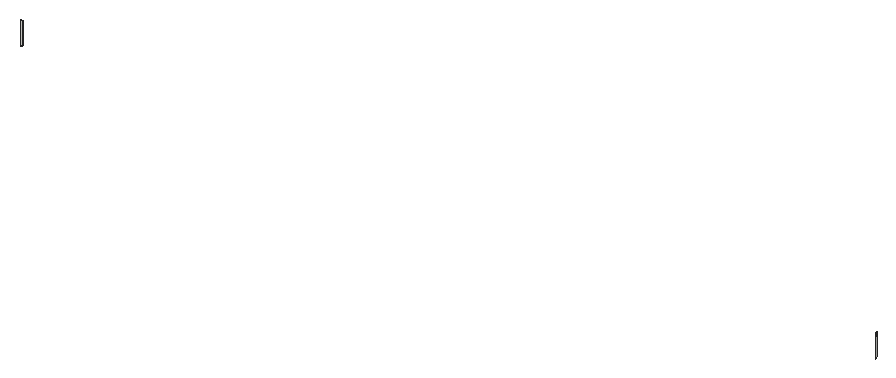
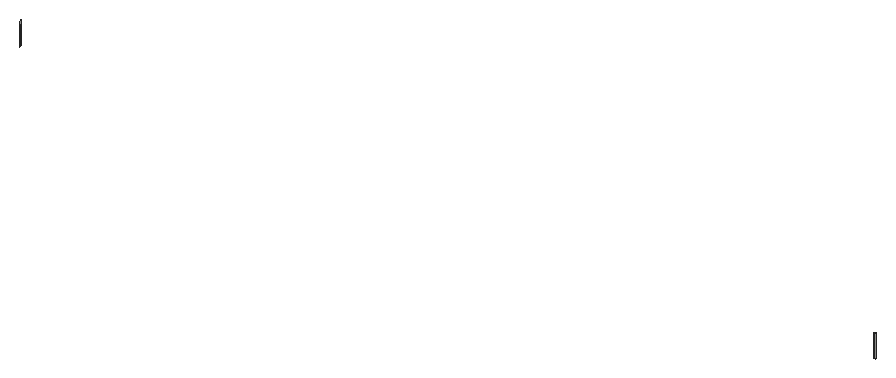
# SketchUp Ruby script. Lengths in inches.
U = 1.inch
M = Sketchup.active_model
def pt(a) = Geom::Point3d.new(a.map { |v| v * U })
def face(e, loops, mat)
  f = e.add_face(loops[0].map { |a| pt(a) })
  loops[1..].each { |l| e.add_face(l.map { |a| pt(a) }).erase! }
  f.material = f.back_material = mat if mat
  f
end
# faces: each face lists its corners as indices into pts; further lists are holes
def faces(e, pts, list, mat = nil) = list.each { |f| face(e, (f[0].is_a?(Array) ? f : [f]).map { |l| l.map { |i| pts[i] } }, mat) }
# xy, xz, yz: faces in a plane at the given z, y or x. An outline is a flat list of corners, or four numbers for a rectangle; further outlines are holes
def ring(l) = l.size == 4 ? [[l[0], l[1]], [l[2], l[1]], [l[2], l[3]], [l[0], l[3]]] : l.each_slice(2).to_a
def flat(e, list, mat, &to3) = list.each { |f| face(e, (f[0].is_a?(Array) ? f : [f]).map { |l| ring(l).map { |u, v| to3.(u, v) } }, mat) }
def xy(e, z, list, mat = nil) = flat(e, list, mat) { |x, y| [x, y, z] }
def xz(e, y, list, mat = nil) = flat(e, list, mat) { |x, z| [x, y, z] }
def yz(e, x, list, mat = nil) = flat(e, list, mat) { |y, z| [x, y, z] }
def lines(e, pts, list) = list.each { |a, b| e.add_line(pt(pts[a]), pt(pts[b])) }
# prism: a flat outline (further loops are holes) pulled along v
def prism(e, loops, v, mat = nil)
  f = face(e, loops, mat); d = Geom::Vector3d.new(v.map { |x| x * U })
  f.pushpull(f.normal.samedirection?(d) ? d.length : -d.length)
end
def box(e, o, s, mat = nil) = prism(e, [[o, [o[0] + s[0], o[1], o[2]], [o[0] + s[0], o[1] + s[1], o[2]], [o[0], o[1] + s[1], o[2]]]], [0, 0, s[2]], mat)
def at(x, y, z, deg = 0) = Geom::Transformation.translation(pt([x, y, z])) * Geom::Transformation.rotation(ORIGIN, Z_AXIS, deg.degrees)
def axes(o, x, y, z) = Geom::Transformation.new([*x, 0, *y, 0, *z, 0, *pt(o).to_a, 1])
def part(name) = M.definitions.add(name)
# library, detail: a bought-in or finely detailed component or shape, given as its bounding box
def library(name, o, s) = part(name).tap { |d| box(d.entities, o, s) }
def detail(e, o, s) = box(e.add_group.entities, o, s)
def put(e, d, t, mat = nil) = e.add_instance(d, t).tap { |i| i.material = mat if mat }
def group(e, t, mat = nil) = e.add_group.tap { |g| g.transformation = t; g.material = mat if mat }.entities
root = M.entities
p = [[215.51,317.21,231],[215.43,317.18,231],[215.43,317.18,234],[215.51,317.21,234],[215.58,317.24,231],[215.58,317.24,234],
  [215.65,317.27,231],[215.65,317.27,234],[215.72,317.31,231],[215.72,317.31,234],[326.84,320.96,231],[326.87,320.88,231],
  [326.87,320.88,234],[326.84,320.96,234],[326.82,321.03,231],[326.82,321.03,234],[326.79,321.11,231],[326.79,321.11,234]]
faces(root,p,[[0,1,2,3],[4,0,3,5],[6,4,5,7],[8,6,7,9],[10,11,12,13],[14,10,13,15],[16,14,15,17]])
